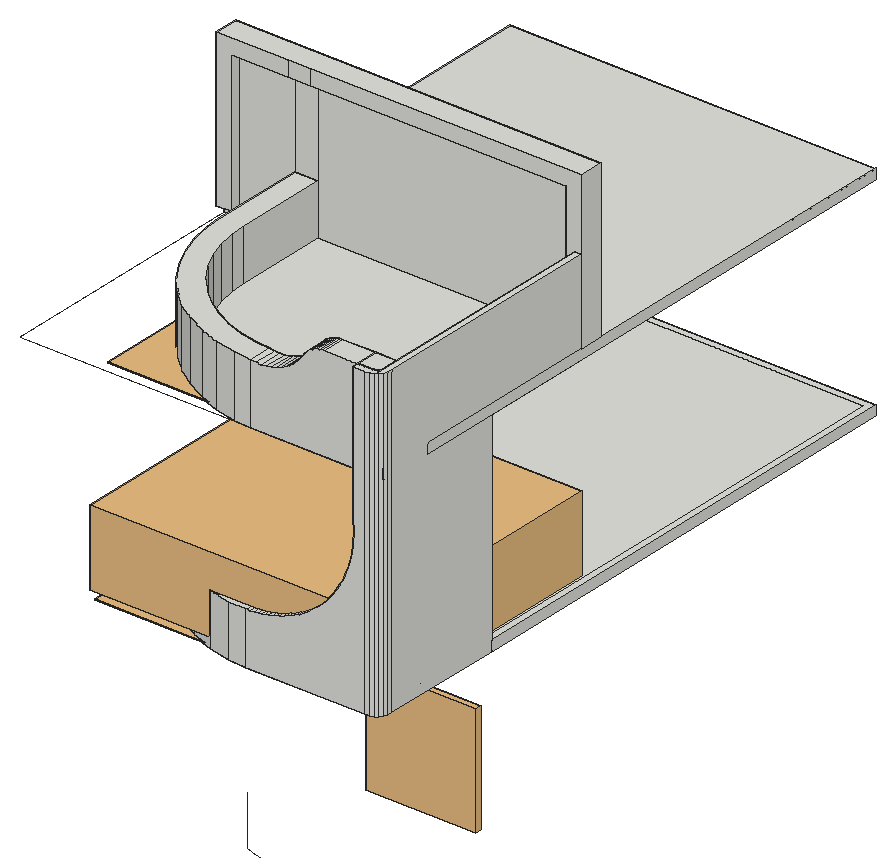
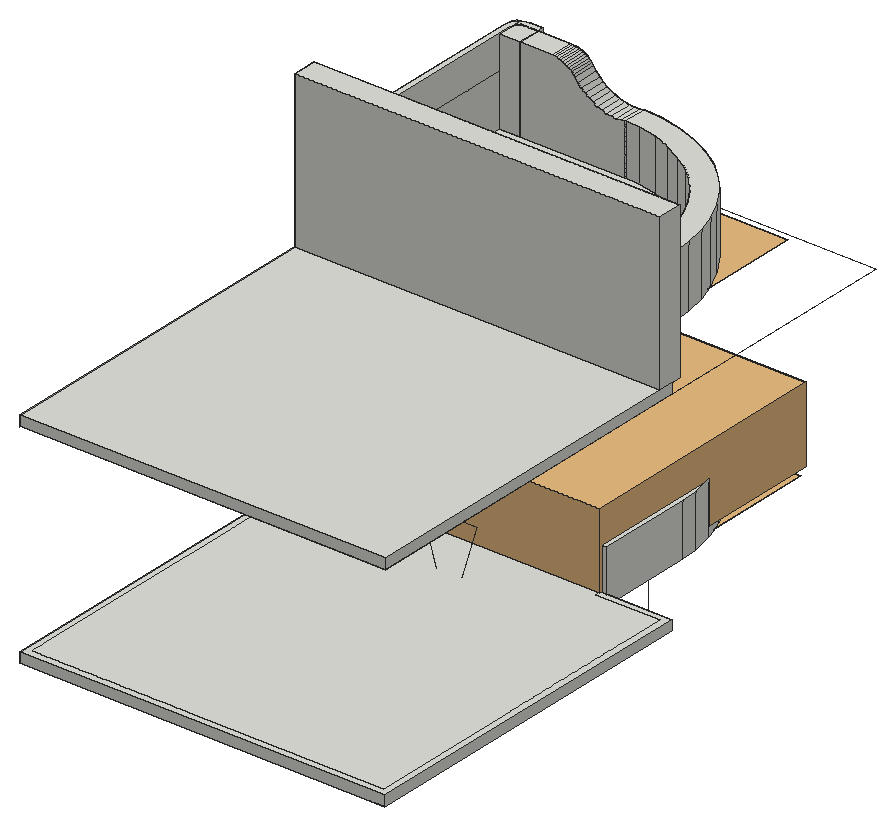
# SketchUp Ruby script. Lengths in inches.
U = 1.inch
M = Sketchup.active_model
def pt(a) = Geom::Point3d.new(a.map { |v| v * U })
def face(e, loops, mat)
  f = e.add_face(loops[0].map { |a| pt(a) })
  loops[1..].each { |l| e.add_face(l.map { |a| pt(a) }).erase! }
  f.material = f.back_material = mat if mat
  f
end
# faces: each face lists its corners as indices into pts; further lists are holes
def faces(e, pts, list, mat = nil) = list.each { |f| face(e, (f[0].is_a?(Array) ? f : [f]).map { |l| l.map { |i| pts[i] } }, mat) }
# xy, xz, yz: faces in a plane at the given z, y or x. An outline is a flat list of corners, or four numbers for a rectangle; further outlines are holes
def ring(l) = l.size == 4 ? [[l[0], l[1]], [l[2], l[1]], [l[2], l[3]], [l[0], l[3]]] : l.each_slice(2).to_a
def flat(e, list, mat, &to3) = list.each { |f| face(e, (f[0].is_a?(Array) ? f : [f]).map { |l| ring(l).map { |u, v| to3.(u, v) } }, mat) }
def xy(e, z, list, mat = nil) = flat(e, list, mat) { |x, y| [x, y, z] }
def xz(e, y, list, mat = nil) = flat(e, list, mat) { |x, z| [x, y, z] }
def yz(e, x, list, mat = nil) = flat(e, list, mat) { |y, z| [x, y, z] }
def lines(e, pts, list) = list.each { |a, b| e.add_line(pt(pts[a]), pt(pts[b])) }
# prism: a flat outline (further loops are holes) pulled along v
def prism(e, loops, v, mat = nil)
  f = face(e, loops, mat); d = Geom::Vector3d.new(v.map { |x| x * U })
  f.pushpull(f.normal.samedirection?(d) ? d.length : -d.length)
end
def box(e, o, s, mat = nil) = prism(e, [[o, [o[0] + s[0], o[1], o[2]], [o[0] + s[0], o[1] + s[1], o[2]], [o[0], o[1] + s[1], o[2]]]], [0, 0, s[2]], mat)
def at(x, y, z, deg = 0) = Geom::Transformation.translation(pt([x, y, z])) * Geom::Transformation.rotation(ORIGIN, Z_AXIS, deg.degrees)
def axes(o, x, y, z) = Geom::Transformation.new([*x, 0, *y, 0, *z, 0, *pt(o).to_a, 1])
def part(name) = M.definitions.add(name)
# library, detail: a bought-in or finely detailed component or shape, given as its bounding box
def library(name, o, s) = part(name).tap { |d| box(d.entities, o, s) }
def detail(e, o, s) = box(e.add_group.entities, o, s)
def put(e, d, t, mat = nil) = e.add_instance(d, t).tap { |i| i.material = mat if mat }
def group(e, t, mat = nil) = e.add_group.tap { |g| g.transformation = t; g.material = mat if mat }.entities
root = M.entities
c1 = library("CTS_Window_Frame\#1",[1571.59,0.98,78.15],[65,4,66])
c2 = part("Group318\#1")
p = [[0,0,0],[0,0,-89.62],[-16.59,0,-89.62],[107.99,-182.15,0],[-107.99,-182.15,0],[107.99,182.15,0],
  [107.99,0,0],[-107.99,182.15,0],[16.59,0,-89.62],[-107.99,0,0],[0,0,-145.07]]
lines(c2.entities,p,[[0,1],[1,2],[3,4],[5,6],[7,5],[1,8],[9,0],[0,6],[8,10],[4,9],[6,3],[2,10],
  [9,7]])
c3 = part("Rectangle Light\#1")
put(c3.entities,c2,at(0,0,0))
c4 = library("Group\#8",[-0.5,-0.5,-0.1],[168.69,156.49,0.2])
c5 = library("Glass Railing\#2",[-169.4375,-0.78,0],[169.99,153.05,35.5])
c6 = library("Group\#9",[-0.5,-0.5,-0.1],[163.58,152.49,0.2])
xy(root,252,[[213.23,54.54,217.23,59.29]])
xz(root,36.44,[[137.85,252,137.85,282.34,138.31,282.28,138.31,252]])
xz(root,54.54,[[213.23,246,217.23,252]])
yz(root,217.23,[[54.54,246,387.4,252]])
p = [[129.46,37.02,252],[129.46,37.02,282.34],[137.85,36.44,282.34],[137.85,36.44,252],[42.64,174.49,126],[38.64,174.49,126],
  [217.23,101.98,126],[217.23,101.98,120],[213.23,59.29,246],[213.23,59.29,252],[217.23,59.29,246],[216.07,23,252],
  [216.07,23,246],[215.89,22.65,252],[216.07,22.65,252],[216.07,22.65,246],[215.89,22.65,246],[132.2,27,18.125],
  [132.2,27,48],[135.3,27,16.91],[139.9,27,15.91]]
faces(root,p,[[0,1,2,3]])
lines(root,p,[[4,5],[6,7],[8,9],[8,10],[11,12],[13,14],[15,16],[14,15],[16,13],[17,18],[17,19],[19,20]])
put(root,c1,at(-1431.22,103.77,-60.22))
put(root,c3,axes([108.21,204.89,245.99],[1,0,0],[0,-1,0],[0,0,1]))
g1 = group(root,at(33.625,101.98,120))
xy(g1,0,[[[104.1,-82.98,93.5,-82.29,80.42,-79.6875,67.79,-75.4,55.83,-69.5,44.74,-62.09,34.71,-53.29,25.91,-43.26,18.5,-32.17,12.6,-20.21,8.3125,-7.58,5.71,5.5,5.02,16.1,5.02,72.51,0,72.51,0,285.41,183.6,285.41,183.6,-73.79,183.34,-76.6,182.58,-78.9,181.3,-80.68,179.51,-81.96,177.21,-82.73,174.4,-82.98],[104.31,-76.54,174.11,-76.54,175.88,-76.375,176.55,-76.15,176.68,-76.0625,176.77,-75.9375,176.99,-75.27,177.15,-73.49,177.15,0,178.15,0,178.15,279.97,5.45,279.97,5.45,77.95,11.46,77.95,11.46,16.31,12.12,6.35,14.55,-5.91,18.57,-17.74,24.09,-28.94,31.04,-39.33,39.27,-48.73,48.67,-56.96,59.06,-63.91,70.26,-69.43,82.09,-73.45,94.35,-75.88]],[-33.41,72.51,0,285.41]])
xy(g1,2,[[104.28,-77.54,94.22,-76.88,81.83,-74.42,69.88,-70.36,58.56,-64.77,48.06,-57.76,38.57,-49.43,30.24,-39.94,23.23,-29.44,17.64,-18.12,13.58,-6.17,11.12,6.22,10.46,16.28,10.46,77.95,5.45,77.95,5.45,279.97,178.15,279.97,178.15,-73.54,177.98,-75.47,177.67,-76.4,177.4,-76.78,177.01,-77.05,176.09,-77.36,174.16,-77.54]])
xy(g1,6,[[104.23,-78.98,174.22,-78.98,176.39,-78.79,177.68,-78.36,178.43,-77.82,178.97,-77.06,179.4,-75.77,179.6,-73.61,179.6,281.41,-29.41,281.41,-29.41,76.51,9.02,76.51,9.02,16.23,9.69,6.03,12.19,-6.54,16.3,-18.68,21.97,-30.17,29.09,-40.82,37.54,-50.46,47.18,-58.91,57.83,-66.03,69.32,-71.7,81.46,-75.81,94.03,-78.31],[179.6,0,183.6,0,183.6,285.41,-33.41,285.41,-33.41,72.51,9.02,72.51,9.02,76.51,-29.41,76.51,-29.41,281.41,179.6,281.41]])
xy(g1,31.08,[[104.1,-82.98,104.25,-82.98,104.25,-78.98,104.23,-78.98,94.03,-78.31,81.46,-75.81,69.32,-71.7,57.83,-66.03,47.18,-58.91,37.54,-50.46,29.09,-40.82,21.97,-30.17,16.3,-18.68,12.19,-6.54,9.69,6.03,9.02,16.23,9.02,72.51,5.02,72.51,5.02,16.1,5.71,5.5,8.3125,-7.58,12.6,-20.21,18.5,-32.17,25.91,-43.26,34.71,-53.29,44.74,-62.09,55.83,-69.5,67.79,-75.4,80.42,-79.6875,93.5,-82.29]])
xy(g1,126,[[179.6,0,183.6,66.69]])
xy(g1,182.34,[[167.23,-82.98,174.4,-82.98,177.21,-82.73,179.51,-81.96,181.3,-80.68,182.58,-78.9,183.34,-76.6,183.6,-73.79,183.6,66.69,179.6,66.69,179.6,-73.61,179.4,-75.77,178.97,-77.06,178.43,-77.82,177.68,-78.36,176.39,-78.79,174.22,-78.98,167.23,-78.98]])
xz(g1,-82.98,[[104.1,0,174.4,0,174.4,182.34,167.23,182.34,167.23,104,167.51,101.83,167.71,99.66,167.84,97.47,167.9,95.29,167.88,93.1,167.79,90.92,167.62,88.74,167.38,86.57,167.0625,84.41,166.67,82.26,166.2,80.12,165.67,78,165.06,75.9,164.375,73.83,163.62,71.78,162.8,69.75,161.91,67.76,160.95,65.79,159.92,63.86,158.83,61.97,157.67,60.12,156.45,58.3,155.17,56.53,153.83,54.81,152.43,53.13,150.97,51.5,149.46,49.92,147.89,48.39,146.28,46.92,144.61,45.51,142.9,44.15,141.14,42.85,139.33,41.62,137.49,40.45,135.61,39.34,133.6875,38.29,131.73,37.32,129.74,36.41,127.73,35.56,125.68,34.79,123.61,34.09,121.52,33.46,119.4,32.91,117.27,32.42,115.125,32.01,112.97,31.68,110.8,31.41,108.62,31.23,106.4375,31.11,104.25,31.08,104.1,31.08]])
xz(g1,-78.98,[[104.23,6,104.23,31.08,104.25,31.08,106.4375,31.11,108.62,31.23,110.8,31.41,112.97,31.68,115.125,32.01,117.27,32.42,119.4,32.91,121.52,33.46,123.61,34.09,125.68,34.79,127.73,35.56,129.74,36.41,131.73,37.32,133.6875,38.29,135.61,39.34,137.49,40.45,139.33,41.62,141.14,42.85,142.9,44.15,144.61,45.51,146.28,46.92,147.89,48.39,149.46,49.92,150.97,51.5,152.43,53.13,153.83,54.81,155.17,56.53,156.45,58.3,157.67,60.12,158.83,61.97,159.92,63.86,160.95,65.79,161.91,67.76,162.8,69.75,163.62,71.78,164.375,73.83,165.06,75.9,165.67,78,166.2,80.12,166.67,82.26,167.0625,84.41,167.38,86.57,167.62,88.74,167.79,90.92,167.88,93.1,167.9,95.29,167.84,97.47,167.71,99.66,167.51,101.83,167.23,104,167.23,162.34,174.22,162.34,174.22,6],[167.23,162.34,174.22,182.34]])
xz(g1,-77.54,[[104.28,1,174.16,2]])
xz(g1,-76.54,[[104.31,0,174.11,1]])
xz(g1,0,[[177.15,0,178.15,1],[179.6,6,183.6,31.08],[179.6,31.08,183.6,104],[179.6,104,183.6,126]])
xz(g1,66.69,[[179.6,126,183.6,182.34]])
xz(g1,72.51,[[-33.41,0,5.02,6],[5.02,6,9.02,31.08]])
xz(g1,77.95,[[5.45,0,5.45,2,10.46,2,10.46,1,11.46,1,11.46,0]])
xz(g1,279.97,[[5.45,0,178.15,2]])
xz(g1,285.41,[[-33.41,0,183.6,6]])
yz(g1,-33.41,[[72.51,0,285.41,6]])
yz(g1,5.02,[[16.1,0,72.51,31.08]])
yz(g1,5.45,[[77.95,0,279.97,2]])
yz(g1,9.02,[[16.23,6,72.51,31.08]])
yz(g1,10.46,[[16.28,1,77.95,2]])
yz(g1,11.46,[[16.31,0,77.95,1]])
yz(g1,167.23,[[-82.98,104,-78.98,162.34],[-82.98,162.34,-78.98,182.34]])
yz(g1,177.15,[[-73.49,0,0,1]])
yz(g1,178.15,[[0,0,279.97,2],[-73.54,1,0,2]])
yz(g1,179.6,[[-73.61,6,-73.61,162.34,66.69,162.34,66.69,126,0,126,0,6],[-73.61,162.34,66.69,182.34]])
yz(g1,183.6,[[-73.79,0,0,0,0,126,66.69,126,66.69,182.34,-73.79,182.34],[0,0,285.41,6]])
p = [[104.1,-82.98,31.08],[93.5,-82.29,31.08],[93.5,-82.29,0],[104.1,-82.98,0],[177.21,-82.73,0],[177.21,-82.73,182.34],
  [174.4,-82.98,182.34],[174.4,-82.98,0],[179.51,-81.96,0],[179.51,-81.96,182.34],[80.42,-79.6875,31.08],[80.42,-79.6875,0],
  [181.3,-80.68,0],[181.3,-80.68,182.34],[182.58,-78.9,0],[182.58,-78.9,182.34],[67.79,-75.4,31.08],[67.79,-75.4,0],
  [183.34,-76.6,0],[183.34,-76.6,182.34],[183.6,-73.79,0],[183.6,-73.79,182.34],[94.35,-75.88,0],[94.35,-75.88,1],
  [104.31,-76.54,1],[104.31,-76.54,0],[174.11,-76.54,0],[174.11,-76.54,1],[175.88,-76.375,1],[175.88,-76.375,0],
  [176.55,-76.15,1],[176.55,-76.15,0],[176.68,-76.0625,1],[176.68,-76.0625,0],[176.77,-75.9375,1],[176.77,-75.9375,0],
  [82.09,-73.45,0],[82.09,-73.45,1],[176.99,-75.27,1],[176.99,-75.27,0],[55.83,-69.5,31.08],[55.83,-69.5,0],
  [177.15,-73.49,1],[177.15,-73.49,0],[70.26,-69.43,0],[70.26,-69.43,1],[44.74,-62.09,31.08],[44.74,-62.09,0],
  [59.06,-63.91,0],[59.06,-63.91,1],[48.67,-56.96,0],[48.67,-56.96,1],[34.71,-53.29,31.08],[34.71,-53.29,0],
  [39.27,-48.73,0],[39.27,-48.73,1],[25.91,-43.26,31.08],[25.91,-43.26,0],[31.04,-39.33,0],[31.04,-39.33,1],
  [18.5,-32.17,31.08],[18.5,-32.17,0],[24.09,-28.94,0],[24.09,-28.94,1],[12.6,-20.21,31.08],[12.6,-20.21,0],
  [18.57,-17.74,0],[18.57,-17.74,1],[8.3125,-7.58,31.08],[8.3125,-7.58,0],[14.55,-5.91,0],[14.55,-5.91,1],
  [5.71,5.5,31.08],[5.71,5.5,0],[12.12,6.35,0],[12.12,6.35,1],[5.02,16.1,31.08],[5.02,16.1,0],
  [11.46,16.31,0],[11.46,16.31,1],[104.28,-77.54,2],[104.28,-77.54,1],[94.22,-76.88,1],[94.22,-76.88,2],
  [176.09,-77.36,2],[176.09,-77.36,1],[174.16,-77.54,1],[174.16,-77.54,2],[177.01,-77.05,2],[177.01,-77.05,1],
  [177.4,-76.78,2],[177.4,-76.78,1],[81.83,-74.42,1],[81.83,-74.42,2],[177.67,-76.4,2],[177.67,-76.4,1],
  [177.98,-75.47,2],[177.98,-75.47,1],[178.15,-73.54,2],[178.15,-73.54,1],[69.88,-70.36,1],[69.88,-70.36,2],
  [58.56,-64.77,1],[58.56,-64.77,2],[48.06,-57.76,1],[48.06,-57.76,2],[38.57,-49.43,1],[38.57,-49.43,2],
  [30.24,-39.94,1],[30.24,-39.94,2],[23.23,-29.44,1],[23.23,-29.44,2],[17.64,-18.12,1],[17.64,-18.12,2],
  [13.58,-6.17,1],[13.58,-6.17,2],[11.12,6.22,1],[11.12,6.22,2],[10.46,16.28,1],[10.46,16.28,2],
  [94.03,-78.31,6],[94.03,-78.31,31.08],[104.23,-78.98,31.08],[104.23,-78.98,6],[174.22,-78.98,162.34],[176.39,-78.79,162.34],
  [176.39,-78.79,6],[174.22,-78.98,6],[177.68,-78.36,162.34],[177.68,-78.36,6],[178.43,-77.82,162.34],[178.43,-77.82,6],
  [81.46,-75.81,6],[81.46,-75.81,31.08],[178.97,-77.06,162.34],[178.97,-77.06,6],[179.4,-75.77,162.34],[179.4,-75.77,6],
  [69.32,-71.7,6],[69.32,-71.7,31.08],[179.6,-73.61,162.34],[179.6,-73.61,6],[57.83,-66.03,6],[57.83,-66.03,31.08],
  [47.18,-58.91,6],[47.18,-58.91,31.08],[37.54,-50.46,6],[37.54,-50.46,31.08],[29.09,-40.82,6],[29.09,-40.82,31.08],
  [21.97,-30.17,6],[21.97,-30.17,31.08],[16.3,-18.68,6],[16.3,-18.68,31.08],[12.19,-6.54,6],[12.19,-6.54,31.08],
  [9.69,6.03,6],[9.69,6.03,31.08],[9.02,16.23,6],[9.02,16.23,31.08],[104.25,-82.98,31.08],[106.4375,-82.98,31.11],
  [106.4375,-78.98,31.11],[104.25,-78.98,31.08],[108.62,-82.98,31.23],[108.62,-78.98,31.23],[110.8,-82.98,31.41],[110.8,-78.98,31.41],
  [112.97,-82.98,31.68],[112.97,-78.98,31.68],[115.125,-82.98,32.01],[115.125,-78.98,32.01],[117.27,-82.98,32.42],[117.27,-78.98,32.42],
  [119.4,-82.98,32.91],[119.4,-78.98,32.91],[121.52,-82.98,33.46],[121.52,-78.98,33.46],[123.61,-82.98,34.09],[123.61,-78.98,34.09],
  [125.68,-82.98,34.79],[125.68,-78.98,34.79],[127.73,-82.98,35.56],[127.73,-78.98,35.56],[129.74,-82.98,36.41],[129.74,-78.98,36.41],
  [131.73,-82.98,37.32],[131.73,-78.98,37.32],[133.6875,-82.98,38.29],[133.6875,-78.98,38.29],[135.61,-82.98,39.34],[135.61,-78.98,39.34],
  [137.49,-82.98,40.45],[137.49,-78.98,40.45],[139.33,-82.98,41.62],[139.33,-78.98,41.62],[141.14,-82.98,42.85],[141.14,-78.98,42.85],
  [142.9,-82.98,44.15],[142.9,-78.98,44.15],[144.61,-82.98,45.51],[144.61,-78.98,45.51],[146.28,-82.98,46.92],[146.28,-78.98,46.92],
  [147.89,-82.98,48.39],[147.89,-78.98,48.39],[149.46,-82.98,49.92],[149.46,-78.98,49.92],[150.97,-82.98,51.5],[150.97,-78.98,51.5],
  [152.43,-82.98,53.13],[152.43,-78.98,53.13],[153.83,-82.98,54.81],[153.83,-78.98,54.81],[155.17,-82.98,56.53],[155.17,-78.98,56.53],
  [156.45,-82.98,58.3],[156.45,-78.98,58.3],[157.67,-82.98,60.12],[157.67,-78.98,60.12],[158.83,-82.98,61.97],[158.83,-78.98,61.97],
  [159.92,-82.98,63.86],[159.92,-78.98,63.86],[160.95,-82.98,65.79],[160.95,-78.98,65.79],[161.91,-82.98,67.76],[161.91,-78.98,67.76],
  [162.8,-82.98,69.75],[162.8,-78.98,69.75],[163.62,-82.98,71.78],[163.62,-78.98,71.78],[164.375,-82.98,73.83],[164.375,-78.98,73.83],
  [165.06,-82.98,75.9],[165.06,-78.98,75.9],[165.67,-82.98,78],[165.67,-78.98,78],[166.2,-82.98,80.12],[166.2,-78.98,80.12],
  [166.67,-82.98,82.26],[166.67,-78.98,82.26],[167.0625,-82.98,84.41],[167.0625,-78.98,84.41],[167.38,-82.98,86.57],[167.38,-78.98,86.57],
  [167.62,-82.98,88.74],[167.62,-78.98,88.74],[167.79,-82.98,90.92],[167.79,-78.98,90.92],[167.88,-82.98,93.1],[167.88,-78.98,93.1],
  [167.9,-82.98,95.29],[167.9,-78.98,95.29],[167.84,-82.98,97.47],[167.84,-78.98,97.47],[167.71,-82.98,99.66],[167.71,-78.98,99.66],
  [167.51,-82.98,101.83],[167.51,-78.98,101.83],[167.23,-82.98,104],[167.23,-78.98,104],[174.22,-78.98,182.34],[176.39,-78.79,182.34],
  [177.68,-78.36,182.34],[178.43,-77.82,182.34],[178.97,-77.06,182.34],[179.4,-75.77,182.34],[179.6,-73.61,182.34],[183.6,-52.67,6],
  [179.6,-52.67,6]]
faces(g1,p,[[0,1,2,3],[4,5,6,7],[8,9,5,4],[1,10,11,2],[12,13,9,8],[14,15,13,12],[10,16,17,11],[18,19,15,14],
  [20,21,19,18],[22,23,24,25],[26,27,28,29],[29,28,30,31],[31,30,32,33],[32,34,35,33],[36,37,23,22],[34,38,39,35],
  [16,40,41,17],[38,42,43,39],[44,45,37,36],[40,46,47,41],[48,49,45,44],[50,51,49,48],[46,52,53,47],[54,55,51,50],
  [52,56,57,53],[54,58,59,55],[56,60,61,57],[58,62,63,59],[60,64,65,61],[62,66,67,63],[64,68,69,65],[66,70,71,67],
  [68,72,73,69],[70,74,75,71],[72,76,77,73],[75,74,78,79],[80,81,82,83],[84,85,86,87],[88,89,85,84],[90,91,89,88],
  [83,82,92,93],[94,95,91,90],[96,97,95,94],[98,99,97,96],[93,92,100,101],[101,100,102,103],[103,102,104,105],[105,104,106,107],
  [107,106,108,109],[109,108,110,111],[111,110,112,113],[113,112,114,115],[115,114,116,117],[117,116,118,119],[120,121,122,123],[124,125,126,127],
  [125,128,129,126],[128,130,131,129],[132,133,121,120],[130,134,135,131],[134,136,137,135],[138,139,133,132],[136,140,141,137],[142,143,139,138],
  [144,145,143,142],[146,147,145,144],[148,149,147,146],[150,151,149,148],[152,153,151,150],[154,155,153,152],[156,157,155,154],[158,159,157,156],
  [160,161,162,163],[161,164,165,162],[164,166,167,165],[166,168,169,167],[168,170,171,169],[170,172,173,171],[172,174,175,173],[174,176,177,175],
  [176,178,179,177],[178,180,181,179],[180,182,183,181],[182,184,185,183],[184,186,187,185],[186,188,189,187],[188,190,191,189],[190,192,193,191],
  [192,194,195,193],[194,196,197,195],[196,198,199,197],[198,200,201,199],[200,202,203,201],[202,204,205,203],[204,206,207,205],[206,208,209,207],
  [208,210,211,209],[210,212,213,211],[212,214,215,213],[214,216,217,215],[216,218,219,217],[218,220,221,219],[220,222,223,221],[222,224,225,223],
  [224,226,227,225],[226,228,229,227],[228,230,231,229],[230,232,233,231],[232,234,235,233],[234,236,237,235],[236,238,239,237],[238,240,241,239],
  [240,242,243,241],[242,244,245,243],[244,246,247,245],[246,248,249,247],[248,250,251,249],[250,252,253,251],[252,254,255,253],[254,256,257,255],
  [256,258,259,257],[258,260,261,259],[124,262,263,125],[125,263,264,128],[128,264,265,130],[130,265,266,134],[134,266,267,136],[136,267,268,140]])
lines(g1,p,[[269,270]])
put(g1,c4,at(10.46,-77.54,1))
put(root,c5,axes([211.3,23.625,126],[1,0,0],[0,1,0],[0,0,1.27]))
put(root,c1,at(-1431.22,103.77,65.78))
g2 = group(root,at(0.22,101.63,246))
xy(g2,0,[[[137.63,-78.98,127.43,-78.31,114.86,-75.81,102.73,-71.7,91.24,-66.03,80.58,-58.91,70.95,-50.46,62.5,-40.82,55.38,-30.17,49.71,-18.68,45.59,-6.54,43.09,6.03,42.42,16.23,42.42,72.51,0,72.51,0,285.41,217.01,285.41,217.01,-73.79,216.75,-76.6,215.98,-78.9,215.92,-78.98],[137.86,-71.98,210.01,-71.98,210.01,0.21,211.01,0.21,211.01,279.41,6,279.41,6,78.51,49.42,78.51,49.42,16.46,50.05,6.94,52.37,-4.73,56.19,-15.99,61.45,-26.66,68.0625,-36.55,75.91,-45.5,84.85,-53.34,94.74,-59.95,105.41,-65.21,116.68,-69.04,128.35,-71.36]]])
xy(g2,2,[[137.83,-72.98,128.22,-72.35,116.42,-70.01,105.03,-66.14,94.24,-60.82,84.24,-54.14,75.2,-46.21,67.27,-37.16,60.59,-27.16,55.27,-16.375,51.4,-4.99,49.05,6.8125,48.42,16.43,48.42,78.51,6,78.51,6,279.41,211.01,279.41,211.01,-72.98]])
xy(g2,6,[[200.63,-78.98,213.01,-65.19],[138.09,-65.19,213.01,-65.19,213.01,-42.69,217.01,-42.69,217.01,67.04,208.01,67.04,208.01,72.51,56.21,72.51,56.21,16.68,56.79,7.83,58.94,-2.96,62.48,-13.39,67.35,-23.26,73.46,-32.41,80.72,-40.6875,89,-47.94,98.15,-54.06,108.02,-58.93,118.44,-62.46,129.24,-64.61],[0,67.04,9,72.51],[208.01,67.04,217.01,67.04,217.01,81.51,0,81.51,0,72.51,208.01,72.51],[0,81.51,217.01,285.41]])
xy(g2,36.34,[[137.63,-78.98,137.63,-65.19,136.625,-65.1,129.24,-64.61,118.44,-62.46,108.02,-58.93,98.15,-54.06,89,-47.94,80.72,-40.6875,73.46,-32.41,67.35,-23.26,62.48,-13.39,58.94,-2.96,56.79,7.83,56.21,16.68,56.21,72.51,42.42,72.51,42.42,16.23,43.09,6.03,45.59,-6.54,49.71,-18.68,55.38,-30.17,62.5,-40.82,70.95,-50.46,80.58,-58.91,91.24,-66.03,102.73,-71.7,114.86,-75.81,127.43,-78.31]])
xy(g2,56.34,[[181.16,-78.98,200.63,-65.19],[200.63,-78.98,213.01,-65.19]])
xy(g2,89.29,[[9,67.04,42.42,72.51],[42.42,67.04,56.21,72.51],[56.21,67.04,208.01,72.51]])
xy(g2,98.29,[[0,67.04,217.01,81.51]])
xz(g2,-78.98,[[137.63,0,215.85,0,215.85,6,200.63,6,200.63,56.34,181.16,56.34,179.87,56.29,178.58,56.13,177.31,55.86,176.07,55.49,174.86,55.02,173.69,54.45,172.57,53.79,171.52,53.04,170.53,52.2,169.61,51.28,168.77,50.29,168.01,49.24,166.29,46.88,164.35,44.71,162.21,42.73,159.89,40.98,157.4,39.46,154.78,38.1875,152.04,37.18,149.22,36.45,146.34,35.99,143.43,35.82,140.52,35.94,137.63,36.34],[200.63,6,213.01,56.34]])
xz(g2,-72.98,[[137.83,1,211.01,2]])
xz(g2,-71.98,[[137.86,0,210.01,1]])
xz(g2,-65.19,[[138.09,6,138.09,36.28,140.52,35.94,143.43,35.82,146.34,35.99,149.22,36.45,152.04,37.18,154.78,38.1875,157.4,39.46,159.89,40.98,162.21,42.73,164.35,44.71,166.29,46.88,168.01,49.24,168.77,50.29,169.61,51.28,170.53,52.2,171.52,53.04,172.57,53.79,173.69,54.45,174.86,55.02,176.07,55.49,177.31,55.86,178.58,56.13,179.87,56.29,181.16,56.34,200.63,56.34,200.63,6],[200.63,6,213.01,56.34]])
xz(g2,0.21,[[210.01,0,211.01,1]])
xz(g2,67.04,[[0,6,9,6,9,89.29,42.42,89.29,42.42,98.29,0,98.29],[208.01,6,217.01,6,217.01,98.29,56.21,98.29,56.21,89.29,208.01,89.29],[42.42,89.29,56.21,98.29]])
xz(g2,72.51,[[0,0,42.42,6],[9,6,42.42,89.29],[42.42,6,56.21,36.34],[56.21,6,208.01,89.29],[42.42,36.34,56.21,89.29]])
xz(g2,78.51,[[6,0,6,2,48.42,2,48.42,1,49.42,1,49.42,0]])
xz(g2,81.51,[[0,6,217.01,98.29]])
xz(g2,279.41,[[6,0,211.01,2]])
xz(g2,285.41,[[0,0,217.01,6]])
yz(g2,0,[[72.51,0,285.41,6],[67.04,6,81.51,98.29]])
yz(g2,6,[[78.51,0,279.41,2]])
yz(g2,9,[[67.04,6,72.51,89.29]])
yz(g2,42.42,[[16.23,0,72.51,36.34]])
yz(g2,48.42,[[16.43,1,78.51,2]])
yz(g2,49.42,[[16.46,0,78.51,1]])
yz(g2,56.21,[[16.68,6,72.51,36.34]])
yz(g2,200.63,[[-78.98,6,-65.19,56.34]])
yz(g2,208.01,[[67.04,6,72.51,89.29]])
yz(g2,210.01,[[-71.98,0,0.21,1]])
yz(g2,211.01,[[0.21,0,279.41,1],[-72.98,1,279.41,2]])
yz(g2,213.01,[[-78.98,6,-65.19,56.34]])
yz(g2,217.01,[[67.04,6,81.51,98.29]])
p = [[137.63,-78.98,0],[137.63,-78.98,36.34],[127.43,-78.31,36.34],[127.43,-78.31,0],[114.86,-75.81,36.34],[114.86,-75.81,0],
  [102.73,-71.7,36.34],[102.73,-71.7,0],[128.35,-71.36,0],[128.35,-71.36,1],[137.86,-71.98,1],[137.86,-71.98,0],
  [91.24,-66.03,36.34],[91.24,-66.03,0],[116.68,-69.04,0],[116.68,-69.04,1],[105.41,-65.21,0],[105.41,-65.21,1],
  [80.58,-58.91,36.34],[80.58,-58.91,0],[94.74,-59.95,0],[94.74,-59.95,1],[84.85,-53.34,0],[84.85,-53.34,1],
  [70.95,-50.46,36.34],[70.95,-50.46,0],[75.91,-45.5,0],[75.91,-45.5,1],[62.5,-40.82,36.34],[62.5,-40.82,0],
  [68.0625,-36.55,0],[68.0625,-36.55,1],[55.38,-30.17,36.34],[55.38,-30.17,0],[61.45,-26.66,0],[61.45,-26.66,1],
  [49.71,-18.68,36.34],[49.71,-18.68,0],[56.19,-15.99,0],[56.19,-15.99,1],[45.59,-6.54,36.34],[45.59,-6.54,0],
  [52.37,-4.73,0],[52.37,-4.73,1],[43.09,6.03,36.34],[43.09,6.03,0],[50.05,6.94,0],[50.05,6.94,1],
  [42.42,16.23,36.34],[42.42,16.23,0],[49.42,16.46,0],[49.42,16.46,1],[137.83,-72.98,2],[137.83,-72.98,1],
  [128.22,-72.35,1],[128.22,-72.35,2],[116.42,-70.01,1],[116.42,-70.01,2],[105.03,-66.14,1],[105.03,-66.14,2],
  [94.24,-60.82,1],[94.24,-60.82,2],[84.24,-54.14,1],[84.24,-54.14,2],[75.2,-46.21,1],[75.2,-46.21,2],
  [67.27,-37.16,1],[67.27,-37.16,2],[60.59,-27.16,1],[60.59,-27.16,2],[55.27,-16.375,1],[55.27,-16.375,2],
  [51.4,-4.99,1],[51.4,-4.99,2],[49.05,6.8125,1],[49.05,6.8125,2],[48.42,16.43,1],[48.42,16.43,2],
  [118.44,-62.46,6],[118.44,-62.46,36.34],[129.24,-64.61,36.34],[129.24,-64.61,6],[108.02,-58.93,6],[108.02,-58.93,36.34],
  [98.15,-54.06,6],[98.15,-54.06,36.34],[89,-47.94,6],[89,-47.94,36.34],[80.72,-40.6875,6],[80.72,-40.6875,36.34],
  [73.46,-32.41,6],[73.46,-32.41,36.34],[67.35,-23.26,6],[67.35,-23.26,36.34],[62.48,-13.39,6],[62.48,-13.39,36.34],
  [58.94,-2.96,6],[58.94,-2.96,36.34],[56.79,7.83,6],[56.79,7.83,36.34],[56.21,16.68,6],[56.21,16.68,36.34],
  [140.52,-78.98,35.94],[143.43,-78.98,35.82],[143.43,-65.19,35.82],[140.52,-65.19,35.94],[146.34,-78.98,35.99],[146.34,-65.19,35.99],
  [138.09,-65.19,36.28],[137.63,-65.19,36.34],[149.22,-78.98,36.45],[149.22,-65.19,36.45],[152.04,-78.98,37.18],[152.04,-65.19,37.18],
  [154.78,-78.98,38.1875],[154.78,-65.19,38.1875],[157.4,-78.98,39.46],[157.4,-65.19,39.46],[159.89,-78.98,40.98],[159.89,-65.19,40.98],
  [162.21,-78.98,42.73],[162.21,-65.19,42.73],[164.35,-78.98,44.71],[164.35,-65.19,44.71],[166.29,-78.98,46.88],[166.29,-65.19,46.88],
  [168.01,-78.98,49.24],[168.01,-65.19,49.24],[168.77,-78.98,50.29],[168.77,-65.19,50.29],[169.61,-78.98,51.28],[169.61,-65.19,51.28],
  [170.53,-78.98,52.2],[170.53,-65.19,52.2],[171.52,-78.98,53.04],[171.52,-65.19,53.04],[172.57,-78.98,53.79],[172.57,-65.19,53.79],
  [173.69,-78.98,54.45],[173.69,-65.19,54.45],[174.86,-78.98,55.02],[174.86,-65.19,55.02],[176.07,-78.98,55.49],[176.07,-65.19,55.49],
  [177.31,-78.98,55.86],[177.31,-65.19,55.86],[178.58,-78.98,56.13],[178.58,-65.19,56.13],[179.87,-78.98,56.29],[179.87,-65.19,56.29],
  [181.16,-78.98,56.34],[181.16,-65.19,56.34]]
faces(g2,p,[[0,1,2,3],[3,2,4,5],[5,4,6,7],[8,9,10,11],[7,6,12,13],[14,15,9,8],[16,17,15,14],[13,12,18,19],
  [20,21,17,16],[22,23,21,20],[19,18,24,25],[26,27,23,22],[24,28,29,25],[26,30,31,27],[28,32,33,29],[30,34,35,31],
  [32,36,37,33],[34,38,39,35],[36,40,41,37],[38,42,43,39],[40,44,45,41],[42,46,47,43],[44,48,49,45],[46,50,51,47],
  [52,53,54,55],[55,54,56,57],[57,56,58,59],[59,58,60,61],[61,60,62,63],[63,62,64,65],[65,64,66,67],[67,66,68,69],
  [69,68,70,71],[71,70,72,73],[73,72,74,75],[75,74,76,77],[78,79,80,81],[82,83,79,78],[84,85,83,82],[86,87,85,84],
  [88,89,87,86],[88,90,91,89],[90,92,93,91],[92,94,95,93],[94,96,97,95],[96,98,99,97],[98,100,101,99],[102,103,104,105],
  [103,106,107,104],[1,102,105,108,109],[106,110,111,107],[110,112,113,111],[112,114,115,113],[114,116,117,115],[116,118,119,117],[118,120,121,119],
  [120,122,123,121],[122,124,125,123],[124,126,127,125],[126,128,129,127],[128,130,131,129],[130,132,133,131],[132,134,135,133],[134,136,137,135],
  [136,138,139,137],[138,140,141,139],[140,142,143,141],[142,144,145,143],[144,146,147,145],[146,148,149,147],[148,150,151,149]])
put(g2,c6,at(48.42,-72.98,1))
